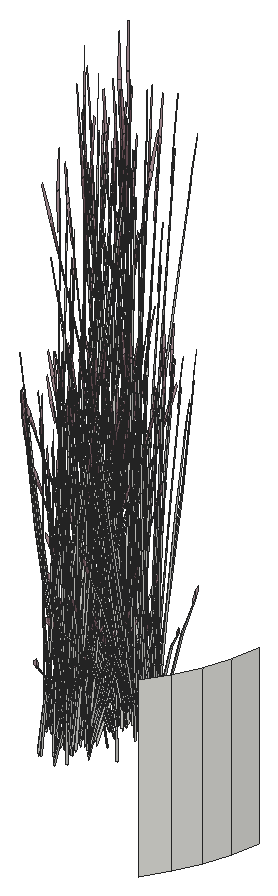
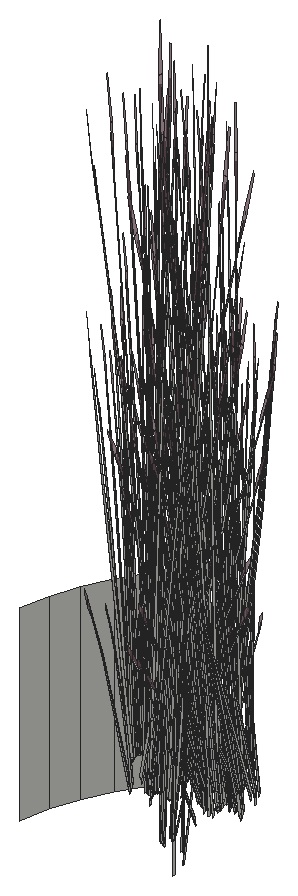
# SketchUp Ruby script. Lengths in inches.
U = 1.inch
M = Sketchup.active_model
def pt(a) = Geom::Point3d.new(a.map { |v| v * U })
def face(e, loops, mat)
  f = e.add_face(loops[0].map { |a| pt(a) })
  loops[1..].each { |l| e.add_face(l.map { |a| pt(a) }).erase! }
  f.material = f.back_material = mat if mat
  f
end
# faces: each face lists its corners as indices into pts; further lists are holes
def faces(e, pts, list, mat = nil) = list.each { |f| face(e, (f[0].is_a?(Array) ? f : [f]).map { |l| l.map { |i| pts[i] } }, mat) }
# xy, xz, yz: faces in a plane at the given z, y or x. An outline is a flat list of corners, or four numbers for a rectangle; further outlines are holes
def ring(l) = l.size == 4 ? [[l[0], l[1]], [l[2], l[1]], [l[2], l[3]], [l[0], l[3]]] : l.each_slice(2).to_a
def flat(e, list, mat, &to3) = list.each { |f| face(e, (f[0].is_a?(Array) ? f : [f]).map { |l| ring(l).map { |u, v| to3.(u, v) } }, mat) }
def xy(e, z, list, mat = nil) = flat(e, list, mat) { |x, y| [x, y, z] }
def xz(e, y, list, mat = nil) = flat(e, list, mat) { |x, z| [x, y, z] }
def yz(e, x, list, mat = nil) = flat(e, list, mat) { |y, z| [x, y, z] }
def lines(e, pts, list) = list.each { |a, b| e.add_line(pt(pts[a]), pt(pts[b])) }
# prism: a flat outline (further loops are holes) pulled along v
def prism(e, loops, v, mat = nil)
  f = face(e, loops, mat); d = Geom::Vector3d.new(v.map { |x| x * U })
  f.pushpull(f.normal.samedirection?(d) ? d.length : -d.length)
end
def box(e, o, s, mat = nil) = prism(e, [[o, [o[0] + s[0], o[1], o[2]], [o[0] + s[0], o[1] + s[1], o[2]], [o[0], o[1] + s[1], o[2]]]], [0, 0, s[2]], mat)
def at(x, y, z, deg = 0) = Geom::Transformation.translation(pt([x, y, z])) * Geom::Transformation.rotation(ORIGIN, Z_AXIS, deg.degrees)
def axes(o, x, y, z) = Geom::Transformation.new([*x, 0, *y, 0, *z, 0, *pt(o).to_a, 1])
def part(name) = M.definitions.add(name)
# library, detail: a bought-in or finely detailed component or shape, given as its bounding box
def library(name, o, s) = part(name).tap { |d| box(d.entities, o, s) }
def detail(e, o, s) = box(e.add_group.entities, o, s)
def put(e, d, t, mat = nil) = e.add_instance(d, t).tap { |i| i.material = mat if mat }
def group(e, t, mat = nil) = e.add_group.tap { |g| g.transformation = t; g.material = mat if mat }.entities
root = M.entities
M.materials.add("LightPink_Translucent").color = [144, 107, 117]
M.materials["LightPink_Translucent"].alpha = 0.75
c1 = part("blade")
p = [[2.15,0.21,22],[0,0.17,0],[0.09,0.45,0],[2.18,0.31,22],[2.29,0.31,22],[0.38,0.45,0],
  [2.48,0.24,33],[2.49,0.24,33],[2.48,0.22,33]]
faces(c1.entities,p,[[0,1,2,3],[4,5,2,3],[6,3,4,7],[8,0,3,6]])
c2 = part("seeds")
p = [[0.3,-0.1,1.38],[-0.01,-0.03,1.59],[-0.01,-0.03,0.03],[0.14,-0.07,-0.07],[0.29,-0.03,3],[0.15,0.01,3.11]]
faces(c2.entities,p,[[0,1,2,3],[1,0,4,5]],"LightPink_Translucent")
c3 = part("blade with seeds")
put(c3.entities,c1,at(0,0,0))
put(c3.entities,c2,axes([2.4,0.25,30.99],[1.5799,-0.05474,1.17369],[-0.12525,1.92788,0.29478],[-0.07173,-0.02425,1.56792]))
p = [[372.76,651.4,618],[371.24,649.12,618],[371.24,649.12,636],[372.76,651.4,636],[373.98,653.86,618],[373.98,653.86,636],
  [374.86,656.47,618],[374.86,656.47,636],[375.4,659.16,618],[375.4,659.16,636]]
faces(root,p,[[0,1,2,3],[4,0,3,5],[6,4,5,7],[8,6,7,9]])
put(root,c3,axes([359.9375,654.26,625.88],[-0.3879,-0.02311,-0.1216],[0.0106,-0.43749,-0.67495],[0.02694,-0.1685,1.02557]))
put(root,c3,axes([360.3,656.16,622.875],[-0.24637,0.29097,-0.30978],[-0.24637,-0.29097,0.30978],[0,0.09372,1.38974]))
put(root,c3,axes([358.34,652.45,622.93],[-0.11756,0.2374,1.1486],[-0.10105,-0.31895,0.84392],[0.09709,-0.07992,0.25299]))
put(root,c3,axes([359.11,660.41,620.59],[-0.10032,0.0944,1.43002],[-0.30046,-0.16522,-0.30754],[0.05569,-0.20547,0.61141]))
put(root,c3,axes([358.2,653.5,624.9],[0.2423,0.19613,0.0643],[-0.14107,0.2793,0.50621],[0.07768,-0.0903,0.77189]))
put(root,c3,axes([361.58,657.48,624.17],[-0.03419,0.06144,1.76342],[-0.3455,0.13246,-0.26939],[-0.08346,-0.12049,0.30037]))
put(root,c3,axes([359.6,656.11,622.94],[0.12941,0.42699,-0.69212],[-0.37279,0.15378,-0.18165],[0.0143,0.14459,1.52773]))
put(root,c3,axes([359.41,655.65,623.05],[0.39487,0,0],[0,0.48281,0],[0,0,1.78407]))
put(root,c3,axes([357.68,661.85,622.98],[0.18436,-0.36797,-0.71045],[0.32306,0.26151,0.08574],[0.11008,-0.13332,1.00501]))
put(root,c3,axes([358.13,653.42,624.9],[0.08753,0.42921,0.48003],[-0.34336,0.07449,0.3958],[0.1012,-0.10094,0.9933]))
put(root,c3,axes([359.79,654.33,625.9],[-0.23881,0.24554,0.35414],[-0.22606,-0.28036,-0.4572],[0.0344,-0.14245,0.87481]))
put(root,c3,axes([359.03,655.12,623.5625],[-0.21202,-0.39143,0.44739],[0.32115,-0.27564,-0.21531],[0.06861,0.04843,1.43643]))
put(root,c3,axes([358.65,655.21,623.51],[-0.04113,-0.53214,-0.29095],[0.42835,-0.03218,-0.50002],[0.07543,-0.07088,1.59708]))
put(root,c3,axes([359.55,655.6,623.46],[0.32884,-0.136,0.1448],[0.11516,0.38837,-0.41347],[0,0.08547,1.26744]))
put(root,c3,axes([359.67,654.1,625.53],[-0.25266,-0.31335,-0.51099],[0.2669,-0.27442,-0.3958],[0.03844,-0.15921,0.97773]))
put(root,c3,axes([357.2,654.7,624.04],[-0.1311,-0.08035,1.71376],[0.27131,-0.33708,0.13857],[0.16909,0.15206,0.73262]))
put(root,c3,axes([358.88,653.49,624.88],[-0.0461,-0.00354,1.77383],[-0.19143,-0.37951,-0.16761],[0.07688,-0.12478,0.31391]))
put(root,c3,axes([359.36,661.11,622.98],[0.00918,-0.43138,-0.71045],[0.38672,0.02897,0.08574],[0.04081,-0.18275,1.00501]))
put(root,c3,axes([359.4375,655.63,623.51],[0.39748,0.22252,-0.29095],[-0.19139,0.46966,-0.50002],[0.01249,0.11531,1.59708]))
put(root,c3,axes([358.17,653.34,624.7],[0.30722,-0.06665,-0.35414],[0.08112,0.381,0.4572],[0.08804,-0.10234,0.87481]))
put(root,c3,axes([357.92,653.46,625.15],[0.18436,-0.36797,-0.71045],[0.32306,0.26151,0.08574],[0.11008,-0.13332,1.00501]))
put(root,c3,axes([358.59,654.03,622.875],[0.32928,0.11539,-0.30978],[-0.08291,0.40636,0.30978],[0.06638,-0.04686,1.38974]))
put(root,c3,axes([358.23,654.59,624.9],[0.12963,0.31798,0.0643],[-0.23638,0.15564,0.50621],[0.1042,-0.03071,0.77189]))
put(root,c3,axes([357.92,655.44,624.7],[0.20082,0.29199,-0.35414],[-0.2293,0.2764,0.4572],[0.1165,0.04206,0.87481]))
put(root,c3,axes([357.69,655.48,625.2],[0.0189,-0.47427,-0.1216],[0.35781,0.01296,-0.67495],[0.13781,0.03295,1.02557]))
put(root,c3,axes([361.36,657.72,624.81],[-0.10181,0.3808,-0.03893],[-0.31336,-0.11714,-0.17649],[-0.04758,-0.06228,0.58215]))
put(root,c3,axes([358.09,654.6,625.2],[-0.17758,-0.42229,-0.1216],[0.31518,-0.20752,-0.67495],[0.13282,-0.05572,1.02557]))
put(root,c3,axes([358.21,654.48,624.9],[-0.09971,0.42522,0.48003],[-0.32782,-0.1454,0.3958],[0.12892,-0.02555,0.9933]))
put(root,c3,axes([362.18,656.43,627.39],[-0.00658,0.0559,1.77383],[-0.32474,0.20287,-0.16761],[-0.09556,-0.1037,0.31391]))
put(root,c3,axes([360.3,655.74,623.32],[0,-0.46636,0.49651],[0.39487,0,0],[0,0.10622,1.57504]))
put(root,c3,axes([360.47,656.17,622.86],[0,0.46636,-0.49651],[-0.39487,0,0],[0,0.10622,1.57504]))
put(root,c3,axes([358.51,653.85,622.86],[0.33032,-0.23318,-0.49651],[0.19744,0.41812,0],[0.07523,-0.05311,1.57504]))
put(root,c3,axes([361.83,657.24,625.27],[-0.02137,0.15256,1.43002],[-0.31245,0.12771,-0.30754],[-0.07303,-0.19719,0.61141]))
put(root,c3,axes([359.18,655.01,623.46],[0.06809,-0.4162,0.1448],[0.33266,0.07225,-0.41347],[0.06054,0.04274,1.26744]))
put(root,c3,axes([361.93,657.63,626.56],[0.08068,0.14973,1.71376],[-0.3728,0.12606,0.13857],[-0.08426,-0.23506,0.73262]))
put(root,c3,axes([359.51,660.85,622.53],[0.23881,-0.24554,-0.35414],[0.22606,0.28036,0.4572],[0.0344,-0.14245,0.87481]))
put(root,c3,axes([362.0625,657.56,627.21],[-0.05451,-0.37564,-0.35414],[0.31161,-0.09919,0.4572],[-0.0837,-0.10765,0.87481]))
put(root,c3,axes([361.2,659.46,625.05],[-0.44133,0,0],[0,-0.52122,-0.51607],[0,-0.11871,1.63711]))
put(root,c3,axes([361.82,660.78,624.71],[-0.08291,-0.40636,-0.30978],[0.32928,-0.11539,0.30978],[-0.06638,-0.04686,1.38974]))
put(root,c3,axes([359.61,660.98,622.73],[0.29004,0.02173,0.0643],[-0.00795,0.32812,0.50621],[0.03035,-0.12569,0.77189]))
put(root,c3,axes([359.65,654.28,623.32],[-0.33032,-0.23318,0.49651],[0.19744,-0.41812,0],[0.07523,0.05311,1.57504]))
put(root,c3,axes([359.75,654.24,625.83],[0.00918,-0.43138,-0.71045],[0.38672,0.02897,0.08574],[0.04081,-0.18275,1.00501]))
put(root,c3,axes([358,655.19,624.88],[0.07571,-0.00789,1.74944],[0.20767,-0.36231,-0.27667],[0.13467,0.04783,0.14031]))
put(root,c3,axes([359.89,660.4375,622.72],[-0.00341,-0.09282,1.74944],[-0.28775,-0.26825,-0.27667],[0.04449,-0.16261,0.14031]))
put(root,c3,axes([359.51,660.95,622.73],[0.25132,0.3182,0.48003],[-0.2669,0.27442,0.3958],[0.04636,-0.14929,0.9933]))
put(root,c3,axes([359.36,656.72,623.03],[0.37054,-0.15823,-0.19198],[0.1302,0.45581,0.00008],[0.0409,-0.01749,1.73897]))
put(root,c3,axes([358.07,654.24,624.85],[0.09562,-0.42421,-0.51099],[0.32782,0.1454,-0.3958],[0.13199,-0.0389,0.97773]))
put(root,c3,axes([358.9,654.51,622.93],[-0.21807,0.07699,1.1486],[0.10265,-0.31819,0.84392],[0.11568,0.02177,0.25299]))
put(root,c3,axes([362.25,657.86,627.73],[0.05451,0.37564,0.35414],[-0.31161,0.09919,-0.4572],[-0.0837,-0.10765,0.87481]))
put(root,c3,axes([358.19,653.125,622.76],[-0.12609,-0.01381,1.43002],[-0.12917,-0.37055,-0.30754],[0.1549,-0.10482,0.61141]))
put(root,c3,axes([361.54,659.32,625.01],[-0.32829,0.39208,0.30756],[-0.32849,-0.38796,-0.36492],[-0.01146,-0.11134,1.64885]))
put(root,c3,axes([359.3,657.33,625.9],[-0.05451,-0.37564,0.35414],[0.31161,-0.09919,-0.4572],[0.0837,0.10765,0.87481]))
put(root,c3,axes([358.28,654.43,624.7],[0.29332,0.1301,-0.35414],[-0.08555,0.37955,0.4572],[0.11809,-0.0348,0.87481]))
put(root,c3,axes([362.89,660.4,626.01],[0.305,0.18805,1.51261],[-0.29879,0.40513,0.59816],[-0.13384,-0.24012,1.26806]))
put(root,c3,axes([359.37,655.36,623.06],[0.21202,0.39143,-0.44739],[-0.32115,0.27564,0.21531],[0.06861,0.04843,1.43643]))
put(root,c3,axes([361.72,656.99,625.45],[0.18411,0.16231,1.1486],[-0.26813,0.09757,0.84392],[-0.05737,-0.12474,0.25299]))
put(root,c3,axes([362.4,659.91,624.89],[-0.21202,-0.39143,-0.44739],[0.32115,-0.27564,0.21531],[-0.06861,-0.04843,1.43643]))
put(root,c3,axes([359.51,655.16,625.32],[-0.30498,-0.24231,1.38283],[0.32203,-0.37727,0.59665],[0.0984,0.22736,1.33663]))
put(root,c3,axes([357.71,655.25,625.15],[0.35281,0.01123,-0.71045],[-0.0237,0.47284,0.08574],[0.14947,0.0499,1.00501]))
put(root,c3,axes([359.91,653.98,625.37],[0.23881,-0.24554,-0.35414],[0.22606,0.28036,0.4572],[0.0344,-0.14245,0.87481]))
put(root,c3,axes([359,657.85,625.55],[0.00104,-0.05646,1.77383],[0.30246,-0.2491,-0.16761],[0.10506,0.08891,0.31391]))
put(root,c3,axes([360,654.11,625.58],[0.29004,0.02173,0.0643],[-0.00795,0.32812,0.50621],[0.03035,-0.12569,0.77189]))
put(root,c3,axes([358.42,654.36,622.15],[-0.22732,0.05597,1.41583],[-0.03618,-0.44548,0.08104],[0.15921,-0.06743,0.80566]))
put(root,c3,axes([359.97,657.14,623.61],[-0.19872,-0.13409,1.1486],[0.2566,-0.13625,0.84392],[0.06921,0.11541,0.25299]))
put(root,c3,axes([358.67,654.07,621.66],[-0.01845,-0.0708,1.76342],[0.12793,-0.41416,-0.26939],[0.12905,-0.00596,0.30037]))
put(root,c3,axes([362.11,657.42,627.77],[0.39316,-0.11987,0.53763],[0.06823,0.47021,0.4433],[-0.09247,-0.13858,1.11249]))
put(root,c3,axes([358.92,660.89,621.875],[-0.06572,0.16029,1.71376],[-0.27569,-0.33172,0.13857],[0.12437,-0.20675,0.73262]))
put(root,c3,axes([360.29,653.57,625.56],[-0.00341,-0.09282,1.74944],[-0.28775,-0.26825,-0.27667],[0.04449,-0.16261,0.14031]))
put(root,c3,axes([358.91,654.8,622.9],[0.23773,-0.35053,-0.62353],[0.29532,0.31785,-0.16365],[0.09526,-0.08744,1.37633]))
put(root,c3,axes([358.8,655.85,624.88],[-0.03191,-0.04083,1.77383],[0.06981,-0.43764,-0.16761],[0.12571,-0.02796,0.31391]))
put(root,c3,axes([359.91,654.08,625.58],[0.25132,0.3182,0.48003],[-0.2669,0.27442,0.3958],[0.04636,-0.14929,0.9933]))
put(root,c3,axes([357.48,653.96,624.04],[-0.14639,0.01056,1.71376],[0.09712,-0.45778,0.13857],[0.20862,0.02831,0.73262]))
put(root,c3,axes([362.2,657.52,627.41],[0.16041,-0.29625,0.0643],[0.22843,0.17248,0.50621],[-0.07385,-0.09498,0.77189]))
put(root,c3,axes([359.96,661.99,623.03],[-0.32648,-0.25715,-0.1216],[0.18809,-0.3724,-0.67495],[0.09224,-0.12945,1.02557]))
put(root,c3,axes([359.95,654.49,622.875],[0.08291,0.40636,-0.30978],[-0.32928,0.11539,0.30978],[0.06638,0.04686,1.38974]))
put(root,c3,axes([360.57,655.82,623.22],[0.44133,0,0],[0,0.52122,-0.51607],[0,0.11871,1.63711]))
put(root,c3,axes([358.01,654.39,625.15],[0.31014,-0.20596,-0.71045],[0.17284,0.42397,0.08574],[0.14985,-0.04816,1.00501]))
put(root,c3,axes([362.43,660.14,625.12],[0.09355,-0.55261,-0.23429],[0.44354,0.09633,0.51271],[-0.0775,-0.07631,1.5644]))
put(root,c3,axes([359.14,655.14,623.51],[0.35635,-0.30962,-0.29095],[0.23697,0.43749,-0.50002],[0.08792,0.04443,1.59708]))
put(root,c3,axes([360.2,655.09,625.9],[-0.30722,0.06665,0.35414],[-0.08112,-0.381,-0.4572],[0.08804,-0.10234,0.87481]))
put(root,c3,axes([359.05,653.9375,624.88],[0.04898,-0.07104,1.74944],[-0.06269,-0.43574,-0.27667],[0.12289,-0.08262,0.14031]))
put(root,c3,axes([362.55,656.64,627.4],[-0.05398,-0.06539,1.74944],[-0.36026,0.04145,-0.27667],[-0.0575,-0.15639,0.14031]))
put(root,c3,axes([359.8125,660.7,619.49],[-0.05283,-0.03674,1.76342],[-0.13569,-0.41045,-0.26939],[0.09154,-0.11138,0.30037]))
put(root,c3,axes([361.29,659.1,624.7],[0,-0.46636,-0.49651],[0.39487,0,0],[0,-0.10622,1.57504]))
put(root,c3,axes([361.46,659.54,625.16],[0,0.46636,0.49651],[-0.39487,0,0],[0,-0.10622,1.57504]))
put(root,c3,axes([359.32,654.02,624.72],[-0.06572,0.16029,1.71376],[-0.27569,-0.33172,0.13857],[0.12437,-0.20675,0.73262]))
put(root,c3,axes([358.49,655.02,622.76],[-0.085,-0.1147,1.43002],[0.1106,-0.37943,-0.30754],[0.17198,0.0514,0.61141]))
put(root,c3,axes([359.8,661.69,622.68],[-0.09067,-0.42583,-0.51099],[0.34336,-0.07449,-0.3958],[0.0984,-0.11438,0.97773]))
put(root,c3,axes([359.27,657.52,625.88],[0.21031,-0.39918,-0.1216],[0.30457,0.22997,-0.67495],[0.10587,0.11278,1.02557]))
put(root,c3,axes([362.33,659.64,625.35],[-0.39748,-0.22252,-0.29095],[0.19139,-0.46966,-0.50002],[-0.01249,-0.11531,1.59708]))
put(root,c3,axes([358.24,654.87,622.4375],[-0.3474,0.18671,1.28929],[-0.11057,-0.53572,0.50096],[0.21332,0.00891,1.46642]))
put(root,c3,axes([360.36,655.12,625.88],[-0.32648,-0.25715,-0.1216],[0.18809,-0.3724,-0.67495],[0.09224,-0.12945,1.02557]))
put(root,c3,axes([362.15,659.17,624.78],[-0.14494,-0.47823,-0.69835],[0.41752,-0.17223,-0.18329],[-0.01602,-0.16194,1.54149]))
put(root,c3,axes([363.1,657.65,627.71],[-0.34538,0.21713,-0.1216],[-0.16972,-0.38536,-0.67495],[-0.04557,-0.16239,1.02557]))
put(root,c3,axes([362.8,657.67,627.36],[-0.34695,-0.11691,-0.51099],[0.11892,-0.40083,-0.3958],[-0.03181,-0.16138,0.97773]))
put(root,c3,axes([359.84,654.04,623.22],[0.22066,-0.46731,0],[0.36918,0.26061,-0.51607],[0.08408,0.05936,1.63711]))
put(root,c3,axes([360.21,653.83,622.34],[-0.05283,-0.03674,1.76342],[-0.13569,-0.41045,-0.26939],[0.09154,-0.11138,0.30037]))
put(root,c3,axes([359.92,656.82,625.9],[-0.20082,-0.29199,0.35414],[0.2293,-0.2764,-0.4572],[0.1165,0.04206,0.87481]))
put(root,c3,axes([360.04,654.32,622.86],[0.33032,0.23318,-0.49651],[-0.19744,0.41812,0],[0.07523,0.05311,1.57504]))
put(root,c3,axes([361.46,659.11,624.71],[0.24637,-0.29097,-0.30978],[0.24637,0.29097,0.30978],[0,-0.09372,1.38974]))
put(root,c3,axes([360.1,657.08,625.58],[-0.01777,0.35463,0.0643],[-0.26836,-0.00972,0.50621],[0.1028,0.03711,0.77189]))
put(root,c3,axes([362.58,657.23,624.81],[-0.2439,0.26754,-0.03893],[-0.22348,-0.29302,-0.17649],[-0.01573,-0.08303,0.58215]))
put(root,c3,axes([360.02,657.64,622.34],[0.02571,-0.06733,1.76342],[0.32373,-0.19829,-0.26939],[0.09815,0.10263,0.30037]))
put(root,c3,axes([360.125,656.97,625.58],[-0.26024,0.30729,0.48003],[-0.22444,-0.32634,0.3958],[0.1221,0.05668,0.9933]))
put(root,c3,axes([360.2,654.82,625.53],[-0.09067,-0.42583,-0.51099],[0.34336,-0.07449,-0.3958],[0.0984,-0.11438,0.97773]))
put(root,c3,axes([362.48,659.87,625.04],[0.44609,0.09826,0.45755],[-0.09078,0.55493,0.17955],[-0.06519,-0.05359,1.58856]))
put(root,c3,axes([360.8,657.02,624.77],[-0.06755,-0.39203,-0.03492],[0.31928,-0.09013,-0.15832],[0.06667,0.02485,0.52218]))
put(root,c3,axes([360.25,656,625.9],[-0.29332,-0.1301,0.35414],[0.08555,-0.37955,-0.4572],[0.11809,-0.0348,0.87481]))
put(root,c3,axes([362.36,659.77,625.4],[-0.17124,0.42022,0.44739],[-0.35581,-0.20224,-0.21531],[0,-0.09687,1.43643]))
put(root,c3,axes([362.93,657.75,627.66],[-0.16845,-0.3792,-0.71045],[0.34676,-0.21133,0.08574],[-0.03939,-0.18322,1.00501]))
put(root,c3,axes([359.56,655.21,622.9],[0.36714,0.07646,-0.62353],[-0.07747,0.47163,-0.16365],[0.10956,0.05715,1.37633]))
put(root,c3,axes([361.12,655.49,623.11],[-0.21881,-0.29821,-0.06488],[0.23965,-0.27324,-0.29416],[0.0679,-0.01924,0.97024]))
put(root,c3,axes([359.8125,661.86,622.98],[0.18436,-0.36797,-0.71045],[0.32306,0.26151,0.08574],[0.11008,-0.13332,1.00501]))
put(root,c3,axes([360.62,653.97,623.61],[-0.11756,0.2374,1.1486],[-0.10105,-0.31895,0.84392],[0.09709,-0.07992,0.25299]))
put(root,c3,axes([360.48,655.03,625.58],[0.2423,0.19613,0.0643],[-0.14107,0.2793,0.50621],[0.07768,-0.0903,0.77189]))
put(root,c3,axes([362.99,657.8,627.73],[-0.1064,0.35863,0.35414],[-0.31043,-0.1046,-0.4572],[-0.02846,-0.14439,0.87481]))
put(root,c3,axes([360.41,654.95,625.58],[0.08753,0.42921,0.48003],[-0.34336,0.07449,0.3958],[0.1012,-0.10094,0.9933]))
put(root,c3,axes([359.48,656.22,624.72],[-0.1311,-0.08035,1.71376],[0.27131,-0.33708,0.13857],[0.16909,0.15206,0.73262]))
put(root,c3,axes([361.16,655.01,625.55],[-0.0461,-0.00354,1.77383],[-0.19143,-0.37951,-0.16761],[0.07688,-0.12478,0.31391]))
put(root,c3,axes([363.1,659.82,624.98],[-0.32829,-0.4014,-0.06131],[0.32849,-0.40164,0],[-0.01146,-0.01402,1.75571]))
put(root,c3,axes([360.45,654.86,625.37],[0.30722,-0.06665,-0.35414],[0.08112,0.381,0.4572],[0.08804,-0.10234,0.87481]))
put(root,c3,axes([360.21,654.99,625.83],[0.18436,-0.36797,-0.71045],[0.32306,0.26151,0.08574],[0.11008,-0.13332,1.00501]))
put(root,c3,axes([360.52,656.12,625.58],[0.12963,0.31798,0.0643],[-0.23638,0.15564,0.50621],[0.1042,-0.03071,0.77189]))
put(root,c3,axes([360.2,656.97,625.37],[0.20082,0.29199,-0.35414],[-0.2293,0.2764,0.4572],[0.1165,0.04206,0.87481]))
put(root,c3,axes([359.97,657,625.88],[0.0189,-0.47427,-0.1216],[0.35781,0.01296,-0.67495],[0.13781,0.03295,1.02557]))
put(root,c3,axes([362.64,656.9,624.17],[-0.0592,0.0168,1.76342],[-0.32738,-0.18913,-0.26939],[0.00549,-0.15776,0.30037]))
put(root,c3,axes([360.375,656.125,625.88],[-0.17758,-0.42229,-0.1216],[0.31518,-0.20752,-0.67495],[0.13282,-0.05572,1.02557]))
put(root,c3,axes([360.49,656,625.58],[-0.09971,0.42522,0.48003],[-0.32782,-0.1454,0.3958],[0.12892,-0.02555,0.9933]))
put(root,c3,axes([362.96,657.42,627.21],[0.1064,-0.35863,-0.35414],[0.31043,0.1046,0.4572],[-0.02846,-0.14439,0.87481]))
put(root,c3,axes([362.4375,659.36,625.04],[0.15345,0.52148,0.45755],[-0.43845,0.18134,0.17955],[0.00536,-0.09582,1.58856]))
put(root,c3,axes([362.37,659.29,624.89],[0.17124,-0.42022,-0.44739],[0.35581,0.20224,0.21531],[0,-0.09687,1.43643]))
put(root,c3,axes([360.29,656.72,625.56],[0.07571,-0.00789,1.74944],[0.20767,-0.36231,-0.27667],[0.13467,0.04783,0.14031]))
put(root,c3,axes([360.36,655.76,625.53],[0.09562,-0.42421,-0.51099],[0.32782,0.1454,-0.3958],[0.13199,-0.0389,0.97773]))
put(root,c3,axes([361.18,656.03,623.61],[-0.21807,0.07699,1.1486],[0.10265,-0.31819,0.84392],[0.11568,0.02177,0.25299]))
put(root,c3,axes([363.09,657.48,627.41],[0.26007,-0.1585,0.0643],[0.12729,0.28902,0.50621],[-0.02512,-0.1274,0.77189]))
put(root,c3,axes([360.47,654.65,623.4375],[-0.12609,-0.01381,1.43002],[-0.12917,-0.37055,-0.30754],[0.1549,-0.10482,0.61141]))
put(root,c3,axes([362.99,659.4,624.89],[0,-0.53961,0],[0.44133,0,0],[0,0,1.79456]))
put(root,c3,axes([363,657.51,627.41],[0.34777,0.12192,0.48003],[-0.11892,0.40083,0.3958],[-0.0209,-0.15763,0.9933]))
put(root,c3,axes([360.56,655.96,625.37],[0.29332,0.1301,-0.35414],[-0.08555,0.37955,0.4572],[0.11809,-0.0348,0.87481]))
put(root,c3,axes([362.58,659.5,625.11],[0.39767,0.22603,0.24065],[-0.19139,0.46966,0.50002],[0,-0.10827,1.60543]))
put(root,c3,axes([362.45,659.1875,625.4],[-0.38326,0.02879,0.44739],[-0.03466,-0.47788,-0.21531],[0.06861,-0.04843,1.43643]))
put(root,c3,axes([359.99,656.78,625.83],[0.35281,0.01123,-0.71045],[-0.0237,0.47284,0.08574],[0.14947,0.0499,1.00501]))
put(root,c3,axes([362.27,658.37,625.15],[-0.10196,0.46348,0.17642],[-0.3731,-0.13116,0.35086],[0.06445,-0.00226,1.60407]))
put(root,c3,axes([360.71,655.88,622.83],[-0.22732,0.05597,1.41583],[-0.03618,-0.44548,0.08104],[0.15921,-0.06743,0.80566]))
put(root,c3,axes([360.96,655.59,622.34],[-0.01845,-0.0708,1.76342],[0.12793,-0.41416,-0.26939],[0.12905,-0.00596,0.30037]))
put(root,c3,axes([361.08,657.38,625.55],[-0.03191,-0.04083,1.77383],[0.06981,-0.43764,-0.16761],[0.12571,-0.02796,0.31391]))
put(root,c3,axes([359.76,655.49,624.72],[-0.14639,0.01056,1.71376],[0.09712,-0.45778,0.13857],[0.20862,0.02831,0.73262]))
put(root,c3,axes([362.09,657.8,625.05],[-0.22066,-0.46731,0],[0.36918,-0.26061,-0.51607],[0.08408,-0.05936,1.63711]))
put(root,c3,axes([360.3,655.92,625.83],[0.31014,-0.20596,-0.71045],[0.17284,0.42397,0.08574],[0.14985,-0.04816,1.00501]))
put(root,c3,axes([363.02,656.67,625.45],[0.04528,0.27194,1.1486],[-0.25117,-0.15062,0.84392],[0.02703,-0.13924,0.25299]))
put(root,c3,axes([362.78,659.0625,625.04],[-0.29264,0.42323,0.45755],[-0.34767,-0.3736,0.17955],[0.07055,-0.04224,1.58856]))
put(root,c3,axes([361.34,655.46,625.56],[0.04898,-0.07104,1.74944],[-0.06269,-0.43574,-0.27667],[0.12289,-0.08262,0.14031]))
put(root,c3,axes([364.09,657.11,627.39],[-0.03584,0.03562,1.77383],[-0.35118,-0.12018,-0.16761],[-0.01271,-0.15545,0.31391]))
put(root,c3,axes([363.82,658.14,627.71],[-0.3879,-0.02311,-0.1216],[0.0106,-0.43749,-0.67495],[0.02694,-0.1685,1.02557]))
put(root,c3,axes([360.77,656.55,623.4375],[-0.085,-0.1147,1.43002],[0.1106,-0.37943,-0.30754],[0.17198,0.0514,0.61141]))
put(root,c3,axes([363.66,658.21,627.73],[-0.23881,0.24554,0.35414],[-0.22606,-0.28036,-0.4572],[0.0344,-0.14245,0.87481]))
put(root,c3,axes([362.91,658.99,625.4],[-0.21202,-0.39143,0.44739],[0.32115,-0.27564,-0.21531],[0.06861,0.04843,1.43643]))
put(root,c3,axes([362.52,659.09,625.35],[-0.04113,-0.53214,-0.29095],[0.42835,-0.03218,-0.50002],[0.07543,-0.07088,1.59708]))
put(root,c3,axes([363.55,657.97,627.36],[-0.25266,-0.31335,-0.51099],[0.2669,-0.27442,-0.3958],[0.03844,-0.15921,0.97773]))
put(root,c3,axes([362.47,657.91,624.71],[0.32928,0.11539,-0.30978],[-0.08291,0.40636,0.30978],[0.06638,-0.04686,1.38974]))
put(root,c3,axes([363.38,657.42,625.27],[-0.10032,0.0944,1.43002],[-0.30046,-0.16522,-0.30754],[0.05569,-0.20547,0.61141]))
put(root,c3,axes([362.39,657.72,624.7],[0.33032,-0.23318,-0.49651],[0.19744,0.41812,0],[0.07523,-0.05311,1.57504]))
put(root,c3,axes([363.05,658.88,625.3],[0.06809,-0.4162,0.1448],[0.33266,0.07225,-0.41347],[0.06054,0.04274,1.26744]))
put(root,c3,axes([363.53,658.16,625.16],[-0.33032,-0.23318,0.49651],[0.19744,-0.41812,0],[0.07523,0.05311,1.57504]))
put(root,c3,axes([363.63,658.12,627.66],[0.00918,-0.43138,-0.71045],[0.38672,0.02897,0.08574],[0.04081,-0.18275,1.00501]))
put(root,c3,axes([363.79,657.86,627.21],[0.23881,-0.24554,-0.35414],[0.22606,0.28036,0.4572],[0.0344,-0.14245,0.87481]))
put(root,c3,axes([363.88,657.98,627.41],[0.29004,0.02173,0.0643],[-0.00795,0.32812,0.50621],[0.03035,-0.12569,0.77189]))
put(root,c3,axes([364.17,657.44,627.4],[-0.00341,-0.09282,1.74944],[-0.28775,-0.26825,-0.27667],[0.04449,-0.16261,0.14031]))
put(root,c3,axes([362.78,658.68,624.74],[0.23773,-0.35053,-0.62353],[0.29532,0.31785,-0.16365],[0.09526,-0.08744,1.37633]))
put(root,c3,axes([363.79,657.95,627.41],[0.25132,0.3182,0.48003],[-0.2669,0.27442,0.3958],[0.04636,-0.14929,0.9933]))
put(root,c3,axes([364.08,658.96,627.73],[-0.30722,0.06665,0.35414],[-0.08112,-0.381,-0.4572],[0.08804,-0.10234,0.87481]))
put(root,c3,axes([363.19,657.9,626.56],[-0.06572,0.16029,1.71376],[-0.27569,-0.33172,0.13857],[0.12437,-0.20675,0.73262]))
put(root,c3,axes([362.12,658.74,624.27],[-0.3474,0.18671,1.28929],[-0.11057,-0.53572,0.50096],[0.21332,0.00891,1.46642]))
put(root,c3,axes([364.24,659,627.71],[-0.32648,-0.25715,-0.1216],[0.18809,-0.3724,-0.67495],[0.09224,-0.12945,1.02557]))
put(root,c3,axes([363.72,657.91,625.06],[0.22066,-0.46731,0],[0.36918,0.26061,-0.51607],[0.08408,0.05936,1.63711]))
put(root,c3,axes([364.09,657.71,624.17],[-0.05283,-0.03674,1.76342],[-0.13569,-0.41045,-0.26939],[0.09154,-0.11138,0.30037]))
put(root,c3,axes([364.08,658.69,627.36],[-0.09067,-0.42583,-0.51099],[0.34336,-0.07449,-0.3958],[0.0984,-0.11438,0.97773]))
put(root,c3,axes([364.125,659.875,627.73],[-0.29332,-0.1301,0.35414],[0.08555,-0.37955,-0.4572],[0.11809,-0.0348,0.87481]))
put(root,c3,axes([365,659.37,624.94],[-0.21881,-0.29821,-0.06488],[0.23965,-0.27324,-0.29416],[0.0679,-0.01924,0.97024]))
put(root,c3,axes([364.5,657.85,625.45],[-0.11756,0.2374,1.1486],[-0.10105,-0.31895,0.84392],[0.09709,-0.07992,0.25299]))
put(root,c3,axes([364.36,658.9,627.41],[0.2423,0.19613,0.0643],[-0.14107,0.2793,0.50621],[0.07768,-0.0903,0.77189]))
put(root,c3,axes([364.29,658.82,627.41],[0.08753,0.42921,0.48003],[-0.34336,0.07449,0.3958],[0.1012,-0.10094,0.9933]))
put(root,c3,axes([365.04,658.89,627.39],[-0.0461,-0.00354,1.77383],[-0.19143,-0.37951,-0.16761],[0.07688,-0.12478,0.31391]))
put(root,c3,axes([364.33,658.74,627.21],[0.30722,-0.06665,-0.35414],[0.08112,0.381,0.4572],[0.08804,-0.10234,0.87481]))
put(root,c3,axes([364.08,658.87,627.66],[0.18436,-0.36797,-0.71045],[0.32306,0.26151,0.08574],[0.11008,-0.13332,1.00501]))
put(root,c3,axes([364.25,660,627.71],[-0.17758,-0.42229,-0.1216],[0.31518,-0.20752,-0.67495],[0.13282,-0.05572,1.02557]))
put(root,c3,axes([364.23,659.64,627.36],[0.09562,-0.42421,-0.51099],[0.32782,0.1454,-0.3958],[0.13199,-0.0389,0.97773]))
put(root,c3,axes([364.35,658.53,625.27],[-0.12609,-0.01381,1.43002],[-0.12917,-0.37055,-0.30754],[0.1549,-0.10482,0.61141]))
put(root,c3,axes([364.58,659.76,624.66],[-0.22732,0.05597,1.41583],[-0.03618,-0.44548,0.08104],[0.15921,-0.06743,0.80566]))
put(root,c3,axes([364.83,659.47,624.17],[-0.01845,-0.0708,1.76342],[0.12793,-0.41416,-0.26939],[0.12905,-0.00596,0.30037]))
put(root,c3,axes([364.17,659.79,627.66],[0.31014,-0.20596,-0.71045],[0.17284,0.42397,0.08574],[0.14985,-0.04816,1.00501]))
put(root,c3,axes([365.21,659.34,627.4],[0.04898,-0.07104,1.74944],[-0.06269,-0.43574,-0.27667],[0.12289,-0.08262,0.14031]))
